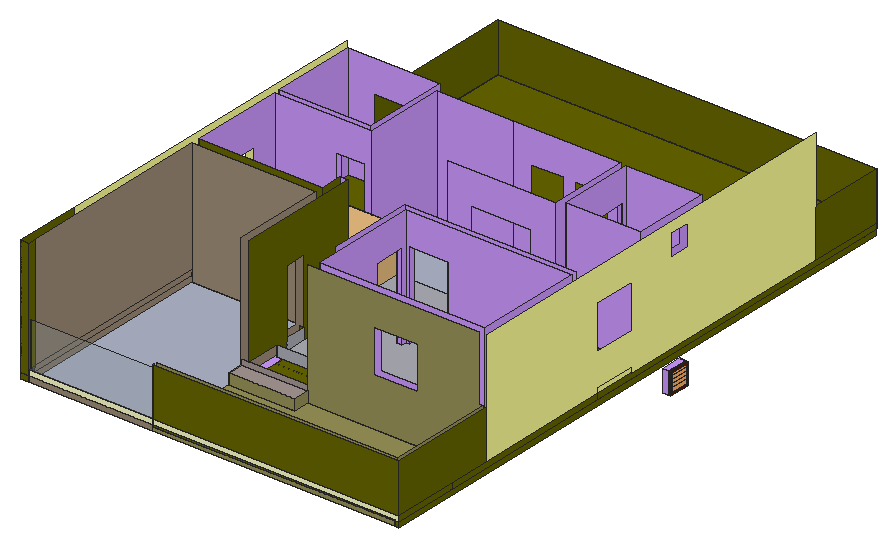
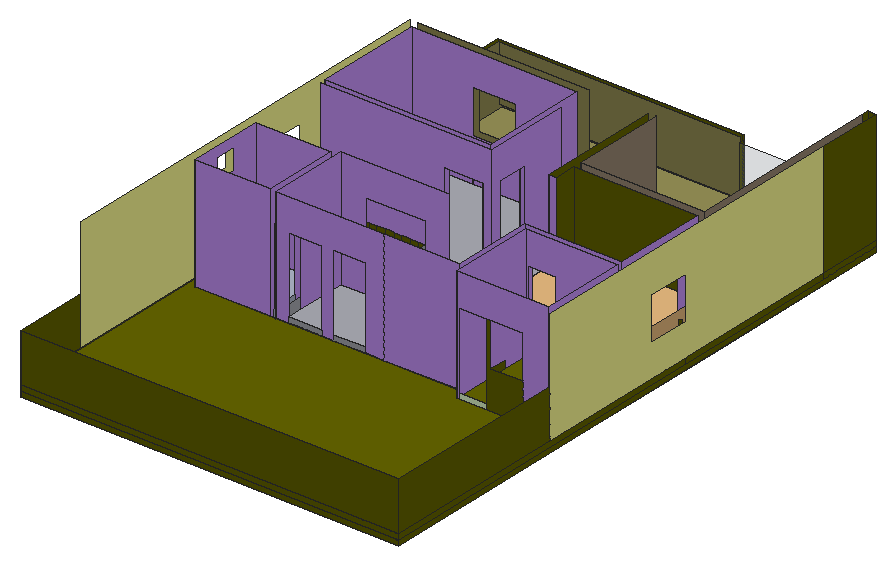
# SketchUp Ruby script. Lengths in inches.
U = 1.inch
M = Sketchup.active_model
def pt(a) = Geom::Point3d.new(a.map { |v| v * U })
def face(e, loops, mat)
  f = e.add_face(loops[0].map { |a| pt(a) })
  loops[1..].each { |l| e.add_face(l.map { |a| pt(a) }).erase! }
  f.material = f.back_material = mat if mat
  f
end
# faces: each face lists its corners as indices into pts; further lists are holes
def faces(e, pts, list, mat = nil) = list.each { |f| face(e, (f[0].is_a?(Array) ? f : [f]).map { |l| l.map { |i| pts[i] } }, mat) }
# xy, xz, yz: faces in a plane at the given z, y or x. An outline is a flat list of corners, or four numbers for a rectangle; further outlines are holes
def ring(l) = l.size == 4 ? [[l[0], l[1]], [l[2], l[1]], [l[2], l[3]], [l[0], l[3]]] : l.each_slice(2).to_a
def flat(e, list, mat, &to3) = list.each { |f| face(e, (f[0].is_a?(Array) ? f : [f]).map { |l| ring(l).map { |u, v| to3.(u, v) } }, mat) }
def xy(e, z, list, mat = nil) = flat(e, list, mat) { |x, y| [x, y, z] }
def xz(e, y, list, mat = nil) = flat(e, list, mat) { |x, z| [x, y, z] }
def yz(e, x, list, mat = nil) = flat(e, list, mat) { |y, z| [x, y, z] }
def lines(e, pts, list) = list.each { |a, b| e.add_line(pt(pts[a]), pt(pts[b])) }
# prism: a flat outline (further loops are holes) pulled along v
def prism(e, loops, v, mat = nil)
  f = face(e, loops, mat); d = Geom::Vector3d.new(v.map { |x| x * U })
  f.pushpull(f.normal.samedirection?(d) ? d.length : -d.length)
end
def box(e, o, s, mat = nil) = prism(e, [[o, [o[0] + s[0], o[1], o[2]], [o[0] + s[0], o[1] + s[1], o[2]], [o[0], o[1] + s[1], o[2]]]], [0, 0, s[2]], mat)
def at(x, y, z, deg = 0) = Geom::Transformation.translation(pt([x, y, z])) * Geom::Transformation.rotation(ORIGIN, Z_AXIS, deg.degrees)
def axes(o, x, y, z) = Geom::Transformation.new([*x, 0, *y, 0, *z, 0, *pt(o).to_a, 1])
def part(name) = M.definitions.add(name)
# library, detail: a bought-in or finely detailed component or shape, given as its bounding box
def library(name, o, s) = part(name).tap { |d| box(d.entities, o, s) }
def detail(e, o, s) = box(e.add_group.entities, o, s)
def put(e, d, t, mat = nil) = e.add_instance(d, t).tap { |i| i.material = mat if mat }
def group(e, t, mat = nil) = e.add_group.tap { |g| g.transformation = t; g.material = mat if mat }.entities
root = M.entities
M.materials.add("B08_Burnt_Sienna").color = [102, 25, 0]
M.materials.add("C03_Honey_Glow").color = [255, 178, 101]
M.materials.add("E01_Mint_Frost").color = [255, 255, 204]
M.materials.add("E02_Pale_Lime").color = [255, 255, 153]
M.materials.add("E08_Lime_Depth").color = [102, 102, 0]
M.materials.add("Glass_Basic_01").color = [161, 173, 186]
M.materials["Glass_Basic_01"].alpha = 0.25
M.materials.add("J02_Lavender_Veil").color = [204, 153, 255]
M.materials.add("Marble_01_1K").color = [230, 255, 211]
M.materials.add("Marble_03_1K").color = [175, 182, 201]
M.materials.add("Marble_06_1K").color = [165, 150, 147]
M.materials.add("Marble_20_1K").color = [172, 173, 182]
M.materials.add("Plaster_02_1K").color = [157, 140, 119]
M.materials.add("Plywood_01_1K").color = [125, 96, 64]
M.materials.add("Soil_04_1K").color = [152, 146, 88]
M.materials.add("Wood_Veneer_15_1K").color = [103, 69, 45]
c1 = part("Group\#58")
xy(c1.entities,0,[[0,0,2.5,24]],"B08_Burnt_Sienna")
xy(c1.entities,1.73,[[1,1.73,2.5,22.27]],"B08_Burnt_Sienna")
xy(c1.entities,1.73,[[0,1.73,1,22.27]],"C03_Honey_Glow")
xy(c1.entities,6.06,[[0,1.73,1,22.27]],"C03_Honey_Glow")
xy(c1.entities,6.54,[[0,1.73,1,22.27]],"C03_Honey_Glow")
xy(c1.entities,10.31,[[0,1.73,1,22.27]],"C03_Honey_Glow")
xy(c1.entities,10.84,[[0,1.73,1,22.27]],"C03_Honey_Glow")
xy(c1.entities,14.12,[[0,1.73,1,22.27]],"C03_Honey_Glow")
xy(c1.entities,14.57,[[0,1.73,1,22.27]],"C03_Honey_Glow")
xy(c1.entities,18.12,[[0,1.73,1,22.27]],"C03_Honey_Glow")
xy(c1.entities,18.66,[[0,1.73,1,22.27]],"C03_Honey_Glow")
xy(c1.entities,22.27,[[1,1.73,2.5,22.27]],"B08_Burnt_Sienna")
xy(c1.entities,22.27,[[0,1.73,1,22.27]],"C03_Honey_Glow")
xy(c1.entities,24,[[0,0,2.5,24]],"B08_Burnt_Sienna")
xz(c1.entities,0,[[0,0,2.5,24]],"B08_Burnt_Sienna")
xz(c1.entities,1.73,[[0,18.12,1,18.66]])
xz(c1.entities,1.73,[[1,1.73,1,6.06,0,6.06,0,6.54,1,6.54,1,10.31,0,10.31,0,10.84,1,10.84,1,14.12,0,14.12,0,14.57,1,14.57,1,22.27,2.5,22.27,2.5,1.73]],"B08_Burnt_Sienna")
xz(c1.entities,1.73,[[0,1.73,1,6.06],[0,6.54,1,10.31],[0,10.84,1,14.12],[0,14.57,1,18.12],[0,18.66,1,22.27]],"C03_Honey_Glow")
xz(c1.entities,22.27,[[0,18.12,1,18.66]])
xz(c1.entities,22.27,[[1,1.73,2.5,1.73,2.5,22.27,1,22.27,1,14.57,0,14.57,0,14.12,1,14.12,1,10.84,0,10.84,0,10.31,1,10.31,1,6.54,0,6.54,0,6.06,1,6.06]],"B08_Burnt_Sienna")
xz(c1.entities,22.27,[[0,1.73,1,6.06],[0,6.54,1,10.31],[0,10.84,1,14.12],[0,14.57,1,18.12],[0,18.66,1,22.27]],"C03_Honey_Glow")
xz(c1.entities,24,[[0,0,2.5,24]],"B08_Burnt_Sienna")
yz(c1.entities,0,[[[0,0,24,24],[1.73,1.73,22.27,22.27]]],"B08_Burnt_Sienna")
yz(c1.entities,0,[[1.73,1.73,22.27,6.06],[1.73,6.54,22.27,10.31],[1.73,10.84,22.27,14.12],[1.73,14.57,22.27,18.12],[1.73,18.66,22.27,22.27]],"C03_Honey_Glow")
yz(c1.entities,1,[[1.73,1.73,22.27,6.06],[1.73,6.54,22.27,10.31],[1.73,10.84,22.27,14.12],[1.73,14.57,22.27,18.12],[1.73,18.66,22.27,22.27]],"C03_Honey_Glow")
yz(c1.entities,2.5,[[[0,0,24,24],[1.73,1.73,22.27,22.27]]],"B08_Burnt_Sienna")
c2 = library("Group\#18",[0,0,-13],[137.375,104.9375,49.125])
c3 = part("Group\#48")
xy(c3.entities,0,[[0,0,73.6875,17.1875]],"Marble_06_1K")
xy(root,120.9375,[[1978.04,2117.58,1987.04,2141.58]],"Plywood_01_1K")
xy(root,135.24,[[1722.42,1900.1875,1788.11,1912.1875]],"Plywood_01_1K")
xy(root,144.9375,[[1978.04,2117.58,1987.04,2141.58]],"J02_Lavender_Veil")
xy(root,156,[[1567.04,1740.42,1567.04,2402.64,1987.04,2401.71,1987.04,1740.42,1982.36,1740.42,1982.36,1862.58,1788.11,1862.58,1788.11,1845.39,1714.42,1845.39,1714.42,1862.58,1713.42,1862.58,1713.42,1967.64,1576.04,1967.64,1576.04,1740.42]],"E08_Lime_Depth")
xy(root,156,[[[1713.42,1862.58,1722.42,1862.58,1722.42,2000.64,1713.42,2000.64,1713.42,1976.64,1576.04,1976.64,1576.04,2081.58,1684.04,2081.58,1684.04,2171.58,1888.04,2171.58,1888.04,2081.58,1978.04,2081.58,1978.04,1997.58,1788.11,1997.58,1788.11,1862.58,1987.04,1862.58,1987.04,2318.58,1678.04,2318.58,1678.04,2192.58,1567.04,2192.58,1567.04,1967.64,1713.42,1967.64],[1794.11,1871.58,1978.04,1991.58],[1684.04,2177.58,1828.04,2309.58],[1834.04,2177.58,1978.04,2309.58],[1576.04,2087.58,1678.04,2183.58],[1894.04,2087.58,1978.04,2171.58]]],"J02_Lavender_Veil")
xy(root,156,[[1576.04,1740.42,1576.04,1967.64,1713.42,1967.64,1713.42,1862.58,1714.42,1862.58,1714.42,1740.42]],"Marble_03_1K")
xy(root,156,[[1567.04,1740.42,1576.04,1967.64],[1722.42,1900.1875,1788.11,1912.1875]],"Plywood_01_1K")
xy(root,156,[[1714.42,1740.42,1714.42,1845.39,1788.11,1845.39,1788.11,1862.58,1982.36,1862.58,1982.36,1740.42]],"Soil_04_1K")
xy(root,160.48,[[1714.42,1740.42,1982.36,1745.11]],"Soil_04_1K")
xy(root,162,[[1567.04,1740.42,1576.04,2005.11],[1576.04,1740.42,1714.42,1745.11],[1567.04,2005.11,1567.04,2402.64,1987.04,2401.71,1987.04,2015.58,1978.04,2015.58,1978.04,2171.58,1684.04,2171.58,1684.04,2087.58,1678.04,2087.58,1678.04,2183.58,1576.04,2183.58,1576.04,2005.11],[1987.04,2401.71,1567.04,2402.64,1987.04,2402.64]],"E08_Lime_Depth")
xy(root,162,[[1600.04,2000.64,1713.42,2000.64,1713.42,2030.95,1675.875,2030.95,1675.875,2081.58,1642.13,2081.58,1642.13,2057.58,1600.04,2057.58],[1576.04,2087.58,1678.04,2183.58]],"Marble_01_1K")
xy(root,162,[[1684.04,2081.58,1768.04,2171.58],[1894.04,2087.58,1978.04,2171.58]],"Marble_03_1K")
xy(root,162,[[[1794.11,1871.58,1978.04,1871.58,1978.04,1991.58,1840.09,1991.58,1840.09,1997.58,1861.04,1997.58,1861.04,2038.58,1940.04,2038.58,1940.04,2040.58,1888.04,2040.58,1888.04,2171.58,1768.04,2171.58,1768.04,2081.58,1675.875,2081.58,1675.875,2030.95,1713.42,2030.95,1713.42,2000.64,1722.42,2000.64,1722.42,1901.49,1788.11,1901.49,1788.11,1951.47,1794.11,1951.47],[1788.11,1985.89,1788.11,1997.58,1798.45,1997.58,1798.45,1991.58,1794.11,1991.58,1794.11,1985.89]]],"Marble_20_1K")
xy(root,168,[[1576.04,1740.42,1714.42,1741.67],[1567.04,1814.64,1576.04,1814.64,1576.04,2087.58,1684.04,2087.58,1684.04,2171.58,1978.04,2171.58,1978.04,2015.58,1987.04,2015.58,1987.04,2402.64,1567.04,2402.64]],"E08_Lime_Depth")
xz(root,1740.42,[[1576.04,162,1714.42,168],[1714.42,162,1987.04,168]],"E01_Mint_Frost")
xz(root,1740.42,[[1567.04,156,1576.04,162],[1982.36,156,1987.04,162],[1714.42,160.48,1982.36,162],[1567.04,162,1576.04,294],[1714.42,168,1987.04,222]],"E08_Lime_Depth")
xz(root,1740.42,[[1576.04,156,1714.42,162]],"Plaster_02_1K")
xz(root,1740.42,[[1714.42,156,1982.36,160.48]],"Soil_04_1K")
xz(root,1745.11,[[1576.04,162,1714.42,216.0625]],"Glass_Basic_01")
xz(root,1745.11,[[1714.42,160.48,1982.36,222]],"Soil_04_1K")
xz(root,1845.39,[[1714.42,156,1788.11,168]],"Soil_04_1K")
xz(root,1862.58,[[1714.42,168,1788.11,168,1788.11,174,1722.42,174,1722.42,174.4375,1714.42,174.4375]],"Marble_06_1K")
xz(root,1862.58,[[1713.42,156,1714.42,168],[1713.42,168,1714.42,294]],"Plaster_02_1K")
xz(root,1862.58,[[[1788.11,156,1788.11,294,1978.04,294,1978.04,222,1982.36,222,1982.36,156],[1862.07,210,1910.07,258]]],"Soil_04_1K")
xz(root,1871.58,[[[1794.11,162,1978.04,294],[1862.07,210,1910.07,258]]],"J02_Lavender_Veil")
xz(root,1900.1875,[[1722.42,135.24,1788.11,156]],"Plywood_01_1K")
xz(root,1901.49,[[1722.42,162,1788.11,174]],"Marble_20_1K")
xz(root,1912.1875,[[1722.42,135.24,1788.11,156]],"Plywood_01_1K")
xz(root,1940.04,[[1717.92,162,1722.42,174]],"E08_Lime_Depth")
xz(root,1951.47,[[1788.11,162,1794.11,258]],"J02_Lavender_Veil")
xz(root,1967.64,[[1576.04,156,1713.42,294]],"Plaster_02_1K")
xz(root,1976.64,[[1576.04,162,1713.42,294]],"E08_Lime_Depth")
xz(root,1985.89,[[1788.11,162,1794.11,258]],"J02_Lavender_Veil")
xz(root,1991.58,[[1794.11,162,1798.45,162,1798.45,258,1840.09,258,1840.09,162,1978.04,162,1978.04,294,1794.11,294]],"J02_Lavender_Veil")
xz(root,1997.58,[[1861.04,162,1870.04,174],[1870.04,162,1879.04,174],[1879.04,162,1888.04,174],[1888.04,162,1897.04,174],[1897.04,162,1906.04,174],
  [1906.04,162,1915.04,174],[1915.04,162,1924.04,174],[1924.04,162,1933.04,174],[1933.04,162,1942.04,174],[1942.04,162,1978.04,174]],"E08_Lime_Depth")
xz(root,1997.58,[[1788.11,162,1788.11,294,1978.04,294,1978.04,174,1861.04,174,1861.04,162,1840.09,162,1840.09,258,1798.45,258,1798.45,162]],"J02_Lavender_Veil")
xz(root,2000.64,[[1713.42,162,1721.79,294],[1721.79,162,1722.42,294]],"J02_Lavender_Veil")
xz(root,2000.64,[[1600.04,162,1713.42,175]],"Wood_Veneer_15_1K")
xz(root,2005.11,[[1571.54,162,1576.04,204]],"E08_Lime_Depth")
xz(root,2015.58,[[1978.04,162,1982.54,168],[1982.54,162,1987.04,168],[1978.04,168,1982.54,174],[1982.54,168,1987.04,174]],"E08_Lime_Depth")
xz(root,2038.58,[[1861.04,162,1940.04,174]],"Marble_20_1K")
xz(root,2040.58,[[1888.04,162,1940.04,174]],"Marble_20_1K")
xz(root,2057.58,[[1600.04,162,1642.13,175]],"Wood_Veneer_15_1K")
xz(root,2081.58,[[1642.13,162,1644.54,162,1644.54,258,1675.875,258,1675.875,162,1684.04,162,1684.04,294,1576.04,294,1576.04,175,1642.13,175],[1768.04,162,1768.04,294,1888.04,294,1888.04,162,1861.04,162,1861.04,258,1794.48,258,1794.48,162]],"J02_Lavender_Veil")
xz(root,2081.58,[[1644.54,162,1675.875,174]],"Marble_01_1K")
xz(root,2087.58,[[1678.04,162,1684.04,168]],"E08_Lime_Depth")
xz(root,2087.58,[[1576.04,162,1644.54,168],[1675.875,162,1678.04,168],[1894.04,162,1978.04,294],[1576.04,168,1576.04,294,1678.04,294,1678.04,168,1675.875,168,1675.875,258,1644.54,258,1644.54,168]],"J02_Lavender_Veil")
xz(root,2087.58,[[1644.54,162,1675.875,168],[1644.54,168,1675.875,174]],"Marble_01_1K")
xz(root,2117.58,[[1978.04,120.9375,1987.04,144.9375]],"J02_Lavender_Veil")
xz(root,2141.58,[[1978.04,120.9375,1987.04,144.9375]],"J02_Lavender_Veil")
xz(root,2171.58,[[1888.04,162,1894.04,168]],"E08_Lime_Depth")
xz(root,2171.58,[[1684.04,162,1768.04,168],[1768.04,162,1788.97,168],[1824.97,162,1837.82,168],[1873.82,162,1888.04,168],[1894.04,162,1978.04,168],
  [1684.04,168,1768.04,294],[1768.04,168,1788.97,168,1788.97,258,1824.97,258,1824.97,168,1837.82,168,1837.82,258,1873.82,258,1873.82,168,1888.04,168,1888.04,294,1768.04,294],[1894.04,168,1978.04,294]],"J02_Lavender_Veil")
xz(root,2171.58,[[1788.97,162,1824.97,168],[1837.82,162,1873.82,168],[1788.97,168,1824.97,174],[1837.82,168,1873.82,174]],"Marble_20_1K")
xz(root,2183.58,[[1605.14,162,1644.54,162,1644.54,258,1641.14,258,1641.14,210,1605.14,210]],"E08_Lime_Depth")
xz(root,2183.58,[[1576.04,162,1605.14,162,1605.14,258,1641.14,258,1641.14,258.0625,1644.54,258.0625,1644.54,258,1675.875,258,1675.875,162,1678.04,162,1678.04,294,1576.04,294]],"J02_Lavender_Veil")
xz(root,2183.58,[[1644.54,162,1675.875,174]],"Marble_01_1K")
xz(root,2402.64,[[1567.04,162,1987.04,168],[1567.04,168,1987.04,222]],"E08_Lime_Depth")
yz(root,1567.04,[[[1814.64,168,2192.58,294],[2005.11,204,2053.11,252]]],"E02_Pale_Lime")
yz(root,1567.04,[[1740.42,156,2402.64,162],[1740.42,162,1814.64,168],[1814.64,162,2005.11,168],[2005.11,162,2402.64,168],[1740.42,168,1814.64,294],
  [2192.58,168,2402.64,222]],"E08_Lime_Depth")
yz(root,1576.04,[[1740.42,162,1745.11,168],[1745.11,162,1749.42,168],[1967.64,162,1976.64,168],[2005.11,162,2087.58,168],[1740.42,168,1740.42,294,1749.42,294,1749.42,168,1745.11,168,1745.11,217.5625,1741.67,217.5625,1741.67,168],
  [1741.67,168,1745.11,216.0625]],"E08_Lime_Depth")
yz(root,1576.04,[[1976.64,162,2005.11,168],[2087.58,162,2183.58,294],[1976.64,168,2005.11,168,2005.11,252,2053.11,252,2053.11,175,2081.58,175,2081.58,294,1976.64,294]],"J02_Lavender_Veil")
yz(root,1576.04,[[1740.42,156,1967.64,162],[1749.42,162,1967.64,168],[1749.42,168,1967.64,294]],"Plaster_02_1K")
yz(root,1600.04,[[2000.64,162,2057.58,175]],"Wood_Veneer_15_1K")
yz(root,1642.13,[[2057.58,162,2081.58,175]],"Wood_Veneer_15_1K")
yz(root,1678.04,[[2117.58,162,2141.58,175.9375]],"E08_Lime_Depth")
yz(root,1678.04,[[2087.58,162,2087.58,294,2183.58,294,2183.58,162,2141.58,162,2141.58,175.9375,2117.58,175.9375,2117.58,162]],"J02_Lavender_Veil")
yz(root,1684.04,[[2117.58,162,2141.58,168],[2117.58,168,2141.58,175.9375]],"E08_Lime_Depth")
yz(root,1684.04,[[2081.58,162,2087.58,162,2087.58,168,2117.58,168,2117.58,175.9375,2141.58,175.9375,2141.58,168,2171.58,168,2171.58,294,2081.58,294],[2087.58,162,2117.58,168],[2141.58,162,2171.58,168]],"J02_Lavender_Veil")
yz(root,1713.42,[[1976.64,162,2000.64,294]],"E08_Lime_Depth")
yz(root,1713.42,[[[1862.58,156,1967.64,294],[1916.04,174,1940.04,246]]],"Plaster_02_1K")
yz(root,1714.42,[[1740.42,162,1745.11,162,1745.11,216.0625,1741.67,216.0625,1741.67,168,1740.42,168],[1740.42,168,1741.67,222]],"E08_Lime_Depth")
yz(root,1714.42,[[1845.39,156,1862.58,168]],"Marble_06_1K")
yz(root,1714.42,[[1740.42,160.48,1745.11,162]],"Soil_04_1K")
yz(root,1722.42,[[1901.49,162,1916.04,162,1916.04,246,1940.04,246,1940.04,162,2000.64,162,2000.64,294,1862.58,294,1862.58,174,1901.49,174]],"E08_Lime_Depth")
yz(root,1722.42,[[1916.04,162,1940.04,174]],"Marble_20_1K")
yz(root,1722.42,[[1900.1875,135.24,1912.1875,156]],"Plywood_01_1K")
yz(root,1788.11,[[1901.49,162,1901.49,294,1997.58,294,1997.58,162,1985.89,162,1985.89,258,1951.47,258,1951.47,162]],"J02_Lavender_Veil")
yz(root,1788.11,[[1900.1875,135.24,1901.49,156],[1901.49,135.24,1912.1875,156]],"Plywood_01_1K")
yz(root,1788.11,[[1845.39,156,1862.58,168]],"Soil_04_1K")
yz(root,1794.11,[[1871.58,162,1951.47,162,1951.47,258,1985.89,258,1985.89,162,1991.58,162,1991.58,294,1871.58,294]],"J02_Lavender_Veil")
yz(root,1798.45,[[1991.58,162,1997.58,258]],"J02_Lavender_Veil")
yz(root,1840.09,[[1991.58,162,1997.58,258]],"J02_Lavender_Veil")
yz(root,1861.04,[[1997.58,162,2036.58,174],[2036.58,162,2038.58,174]],"Marble_20_1K")
yz(root,1888.04,[[2081.58,162,2081.58,294,2171.58,294,2171.58,162,2167.61,162,2167.61,258,2137.61,258,2137.61,162]],"J02_Lavender_Veil")
yz(root,1888.04,[[2040.58,162,2042.58,174],[2042.58,162,2081.58,174],[2137.61,162,2167.61,174]],"Marble_20_1K")
yz(root,1894.04,[[2087.58,162,2137.61,162,2137.61,258,2167.61,258,2167.61,162,2171.58,162,2171.58,294,2087.58,294]],"J02_Lavender_Veil")
yz(root,1894.04,[[2137.61,162,2167.61,174]],"Marble_03_1K")
yz(root,1910.07,[[1867.08,162,1871.58,174]],"E08_Lime_Depth")
yz(root,1940.04,[[2038.58,162,2040.58,174]],"Marble_20_1K")
yz(root,1978.04,[[1997.58,162,2015.58,174],[2015.58,162,2087.58,168]],"E08_Lime_Depth")
yz(root,1978.04,[[1871.58,162,1991.58,294],[2087.58,162,2171.58,168],[[2087.58,168,2171.58,294],[2117.58,258.9375,2141.58,282.9375]]],"J02_Lavender_Veil")
yz(root,1982.36,[[1740.42,156,1862.58,156,1862.58,222,1745.11,222,1745.11,160.48,1740.42,160.48]],"Soil_04_1K")
yz(root,1987.04,[[[1862.58,168,2015.58,168,2015.58,174,2063.58,174,2063.58,168,2318.58,168,2318.58,294,1862.58,294],[2015.58,210,2063.58,258.04],[2117.58,258.9375,2141.58,282.9375]],[2015.58,168,2063.58,174]],"E02_Pale_Lime")
yz(root,1987.04,[[1740.42,156,2401.71,162],[1740.42,162,1814.64,168],[1814.64,162,2015.58,168],[2015.58,162,2402.64,168],[1740.42,168,1862.58,222],
  [2318.58,168,2402.64,222]],"E08_Lime_Depth")
p = [[1567.04,2402.64,162],[1987.04,2401.71,162],[1987.04,2401.71,156],[1567.04,2402.64,156],[1978.04,2063.58,168],[1978.04,2063.58,174],
  [1987.04,1814.64,168],[1978.04,1814.64,168]]
faces(root,p,[[0,1,2,3]],"E08_Lime_Depth")
lines(root,p,[[4,5],[6,7]])
put(root,c1,at(1984.54,2117.58,120.9375),"E02_Pale_Lime")
put(root,c2,at(1576.04,1976.64,175),"E08_Lime_Depth")
put(root,c3,at(1714.42,1845.39,168),"E08_Lime_Depth")
